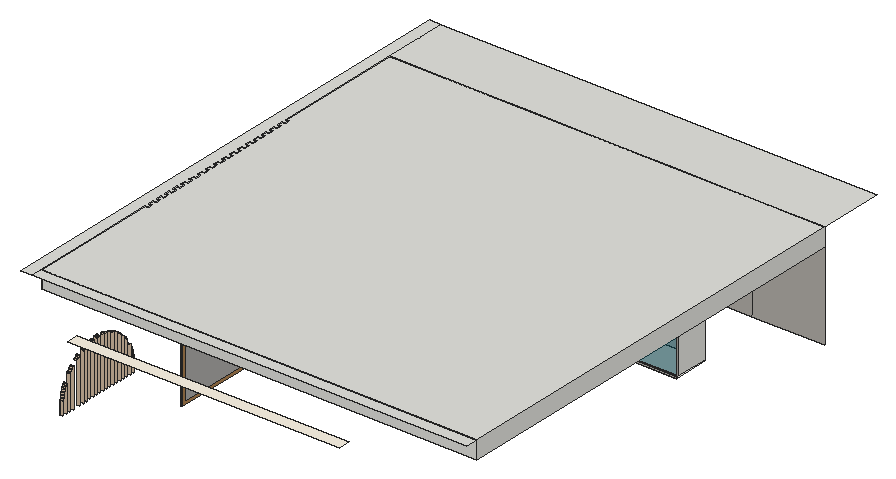
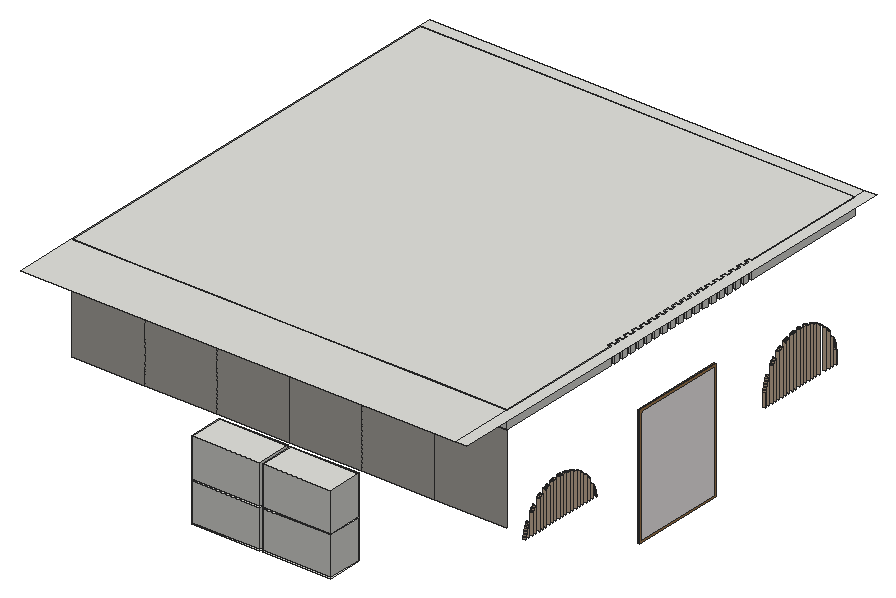
# SketchUp Ruby script. Lengths in inches.
U = 1.inch
M = Sketchup.active_model
def pt(a) = Geom::Point3d.new(a.map { |v| v * U })
def face(e, loops, mat)
  f = e.add_face(loops[0].map { |a| pt(a) })
  loops[1..].each { |l| e.add_face(l.map { |a| pt(a) }).erase! }
  f.material = f.back_material = mat if mat
  f
end
# faces: each face lists its corners as indices into pts; further lists are holes
def faces(e, pts, list, mat = nil) = list.each { |f| face(e, (f[0].is_a?(Array) ? f : [f]).map { |l| l.map { |i| pts[i] } }, mat) }
# xy, xz, yz: faces in a plane at the given z, y or x. An outline is a flat list of corners, or four numbers for a rectangle; further outlines are holes
def ring(l) = l.size == 4 ? [[l[0], l[1]], [l[2], l[1]], [l[2], l[3]], [l[0], l[3]]] : l.each_slice(2).to_a
def flat(e, list, mat, &to3) = list.each { |f| face(e, (f[0].is_a?(Array) ? f : [f]).map { |l| ring(l).map { |u, v| to3.(u, v) } }, mat) }
def xy(e, z, list, mat = nil) = flat(e, list, mat) { |x, y| [x, y, z] }
def xz(e, y, list, mat = nil) = flat(e, list, mat) { |x, z| [x, y, z] }
def yz(e, x, list, mat = nil) = flat(e, list, mat) { |y, z| [x, y, z] }
def lines(e, pts, list) = list.each { |a, b| e.add_line(pt(pts[a]), pt(pts[b])) }
# prism: a flat outline (further loops are holes) pulled along v
def prism(e, loops, v, mat = nil)
  f = face(e, loops, mat); d = Geom::Vector3d.new(v.map { |x| x * U })
  f.pushpull(f.normal.samedirection?(d) ? d.length : -d.length)
end
def box(e, o, s, mat = nil) = prism(e, [[o, [o[0] + s[0], o[1], o[2]], [o[0] + s[0], o[1] + s[1], o[2]], [o[0], o[1] + s[1], o[2]]]], [0, 0, s[2]], mat)
def at(x, y, z, deg = 0) = Geom::Transformation.translation(pt([x, y, z])) * Geom::Transformation.rotation(ORIGIN, Z_AXIS, deg.degrees)
def axes(o, x, y, z) = Geom::Transformation.new([*x, 0, *y, 0, *z, 0, *pt(o).to_a, 1])
def part(name) = M.definitions.add(name)
# library, detail: a bought-in or finely detailed component or shape, given as its bounding box
def library(name, o, s) = part(name).tap { |d| box(d.entities, o, s) }
def detail(e, o, s) = box(e.add_group.entities, o, s)
def put(e, d, t, mat = nil) = e.add_instance(d, t).tap { |i| i.material = mat if mat }
def group(e, t, mat = nil) = e.add_group.tap { |g| g.transformation = t; g.material = mat if mat }.entities
root = M.entities
M.materials.add("F15").color = [172, 171, 168]
M.materials.add("Querkus Oak Naturel Adagio _ Architonic1").color = [173, 130, 81]
M.materials.add("[0010_Snow]").color = [255, 250, 250]
M.materials.add("[0030_OldLace]").color = [253, 245, 230]
M.materials.add("[0052_FloralWhite]").color = [178, 175, 168]
M.materials.add("[0052_FloralWhite]1").color = [255, 250, 240]
M.materials.add("[Formica Laminate Light]").color = [213, 189, 164]
M.materials.add("[Translucent Glass Tinted]").color = [3, 85, 102]
M.materials["[Translucent Glass Tinted]"].alpha = 0.48
c1 = part("F7")
g1 = group(c1.entities,at(0,0,0))
xy(g1,0.5,[[0.5,0.3,18.5,0.6]])
xy(g1,24,[[0.5,0.3,18.5,0.6]])
xz(g1,0.3,[[0.5,0.5,18.5,24]],"F15")
xz(g1,0.6,[[0.5,0.5,18.5,24]],"[0010_Snow]")
yz(g1,0.5,[[0.3,0.5,0.6,24]])
yz(g1,18.5,[[0.3,0.5,0.6,24]])
g2 = group(g1,at(19,0,0),"Querkus Oak Naturel Adagio _ Architonic1")
prism(g2,[[[0,0.6,0],[0,0.6,24.5],[-19,0.6,24.5],[-19,0.6,0]],[[-0.5,0.6,0.5],[-18.5,0.6,0.5],[-18.5,0.6,24],[-0.5,0.6,24]]],[0,-0.6,0])
c2 = library("chandelier1 (1)",[151.15,151.6,16.88],[49.29,55.59,90.46])
xy(root,68.12,[[54.33,152.5,77.5,164],[78.5,152.5,101.67,164]])
xy(root,68.12,[[54.33,152,77.5,152.5],[78.5,152,101.67,152.5]],"[0052_FloralWhite]")
xy(root,68.62,[[54.33,152.5,77.5,164],[78.5,152.5,101.67,164]])
xy(root,68.62,[[54.33,152,77.5,152.5],[78.5,152,101.67,152.5]],"[0052_FloralWhite]")
xy(root,81.31,[[54.33,152.5,77.5,164],[78.5,152.5,101.67,164]])
xy(root,81.31,[[54.33,152,77.5,152.5],[78.5,152,101.67,152.5]],"[0052_FloralWhite]")
xy(root,81.81,[[54.33,152.5,77.5,164],[78.5,152.5,101.67,164]])
xy(root,81.81,[[54.33,152,77.5,152.5],[78.5,152,101.67,152.5]],"[0052_FloralWhite]")
xy(root,95,[[54.33,152.5,77.5,164],[78.5,152.5,101.67,164]])
xy(root,95,[[54.33,152,77.5,152.5],[78.5,152,101.67,152.5]],"[0052_FloralWhite]")
xy(root,101.71,[[4,24.84,5,24.86],[4,29.14,5,29.16],[4,126.84,5,126.86],[4,131.14,5,131.16]],"[Formica Laminate Light]")
xy(root,116.13,[[16.1875,0,108.6875,4]],"[0030_OldLace]")
xy(root,126,[[[4,4,4,48,5,48,5,49.71,4,49.71,4,51.43,5,51.43,5,53.14,4,53.14,4,54.86,5,54.86,5,56.57,4,56.57,4,58.29,5,58.29,5,60,4,60,4,61.71,5,61.71,5,63.43,4,63.43,4,65.14,5,65.14,5,66.86,4,66.86,4,68.57,5,68.57,5,70.29,4,70.29,4,72,5,72,5,73.71,4,73.71,4,75.43,5,75.43,5,77.14,4,77.14,4,78.86,5,78.86,5,80.57,4,80.57,4,82.29,5,82.29,5,84,4,84,4,85.71,5,85.71,5,87.43,4,87.43,4,89.14,5,89.14,5,90.86,4,90.86,4,92.57,5,92.57,5,94.29,4,94.29,4,96,5,96,5,97.71,4,97.71,4,99.43,5,99.43,5,101.14,4,101.14,4,102.86,5,102.86,5,104.57,4,104.57,4,106.29,5,106.29,5,108,4,108,4,152,152,152,152,4],[37.37,36.37,119.63,119.63]]],"[0052_FloralWhite]1")
xy(root,130,[[37.37,36.37,119.63,119.63]],"[0052_FloralWhite]1")
xy(root,132,[[0,0,4,0,4,48,5,48,5,49.71,4,49.71,4,51.43,5,51.43,5,53.14,4,53.14,4,54.86,5,54.86,5,56.57,4,56.57,4,58.29,5,58.29,5,60,4,60,4,61.71,5,61.71,5,63.43,4,63.43,4,65.14,5,65.14,5,66.86,4,66.86,4,68.57,5,68.57,5,70.29,4,70.29,4,72,5,72,5,73.71,4,73.71,4,75.43,5,75.43,5,77.14,4,77.14,4,78.86,5,78.86,5,80.57,4,80.57,4,82.29,5,82.29,5,84,4,84,4,85.71,5,85.71,5,87.43,4,87.43,4,89.14,5,89.14,5,90.86,4,90.86,4,92.57,5,92.57,5,94.29,4,94.29,4,96,5,96,5,97.71,4,97.71,4,99.43,5,99.43,5,101.14,4,101.14,4,102.86,5,102.86,5,104.57,4,104.57,4,106.29,5,106.29,5,108,4,108,4,174,0,174],[4,0,152,4],[4,4,152,4,152,152,4,152,4,108,5,108,5,106.29,4,106.29,4,104.57,5,104.57,5,102.86,4,102.86,4,101.14,5,101.14,5,99.43,4,99.43,4,97.71,5,97.71,5,96,4,96,4,94.29,5,94.29,5,92.57,4,92.57,4,90.86,5,90.86,5,89.14,4,89.14,4,87.43,5,87.43,5,85.71,4,85.71,4,84,5,84,5,82.29,4,82.29,4,80.57,5,80.57,5,78.86,4,78.86,4,77.14,5,77.14,5,75.43,4,75.43,4,73.71,5,73.71,5,72,4,72,4,70.29,5,70.29,5,68.57,4,68.57,4,66.86,5,66.86,5,65.14,4,65.14,4,63.43,5,63.43,5,61.71,4,61.71,4,60,5,60,5,58.29,4,58.29,4,56.57,5,56.57,5,54.86,4,54.86,4,53.14,5,53.14,5,51.43,4,51.43,4,49.71,5,49.71,5,48,4,48],[4,152,152,174]])
xz(root,4,[[4,126,152,132]])
xz(root,12,[[4,84.25,5,88.86]],"[Formica Laminate Light]")
xz(root,13.43,[[4,84.25,5,93.49]],"[Formica Laminate Light]")
xz(root,14.86,[[4,84.25,5,95.8]],"[Formica Laminate Light]")
xz(root,16.29,[[4,84.25,5,97.4375]],"[Formica Laminate Light]")
xz(root,19.14,[[4,84.25,5,99.67]],"[Formica Laminate Light]")
xz(root,20.57,[[4,84.25,5,100.43]],"[Formica Laminate Light]")
xz(root,22,[[4,84.25,5,101.01]],"[Formica Laminate Light]")
xz(root,23.43,[[4,84.25,5,101.43]],"[Formica Laminate Light]")
xz(root,24.86,[[4,84.25,5,101.71]],"[Formica Laminate Light]")
xz(root,26.29,[[4,84.25,5,101.84]],"[Formica Laminate Light]")
xz(root,27.71,[[4,84.25,5,101.84]],"[Formica Laminate Light]")
xz(root,29.14,[[4,84.25,5,101.71]],"[Formica Laminate Light]")
xz(root,30.57,[[4,84.25,5,101.43]],"[Formica Laminate Light]")
xz(root,32,[[4,84.25,5,101.01]],"[Formica Laminate Light]")
xz(root,33.43,[[4,84.25,5,100.43]],"[Formica Laminate Light]")
xz(root,34.86,[[4,84.25,5,99.67]],"[Formica Laminate Light]")
xz(root,36.29,[[4,84.25,5,98.69]],"[Formica Laminate Light]")
xz(root,36.37,[[37.37,126,119.63,130]],"[0052_FloralWhite]1")
xz(root,37.71,[[4,84.25,5,97.4375]],"[Formica Laminate Light]")
xz(root,39.14,[[4,84.25,5,95.8]],"[Formica Laminate Light]")
xz(root,40.57,[[4,84.25,5,93.49]],"[Formica Laminate Light]")
xz(root,42,[[4,84.25,5,88.86]],"[Formica Laminate Light]")
xz(root,48,[[4,126,5,132]])
xz(root,49.71,[[4,126,5,132]])
xz(root,51.43,[[4,126,5,132]])
xz(root,53.14,[[4,126,5,132]])
xz(root,54.86,[[4,126,5,132]])
xz(root,56.57,[[4,126,5,132]])
xz(root,58.29,[[4,126,5,132]])
xz(root,60,[[4,126,5,132]])
xz(root,61.71,[[4,126,5,132]])
xz(root,63.43,[[4,126,5,132]])
xz(root,65.14,[[4,126,5,132]])
xz(root,66.86,[[4,126,5,132]])
xz(root,68.57,[[4,126,5,132]])
xz(root,70.29,[[4,126,5,132]])
xz(root,72,[[4,126,5,132]])
xz(root,73.71,[[4,126,5,132]])
xz(root,75.43,[[4,126,5,132]])
xz(root,77.14,[[4,126,5,132]])
xz(root,78.86,[[4,126,5,132]])
xz(root,80.57,[[4,126,5,132]])
xz(root,82.29,[[4,126,5,132]])
xz(root,84,[[4,126,5,132]])
xz(root,85.71,[[4,126,5,132]])
xz(root,87.43,[[4,126,5,132]])
xz(root,89.14,[[4,126,5,132]])
xz(root,90.86,[[4,126,5,132]])
xz(root,92.57,[[4,126,5,132]])
xz(root,94.29,[[4,126,5,132]])
xz(root,96,[[4,126,5,132]])
xz(root,97.71,[[4,126,5,132]])
xz(root,99.43,[[4,126,5,132]])
xz(root,101.14,[[4,126,5,132]])
xz(root,102.86,[[4,126,5,132]])
xz(root,104.57,[[4,126,5,132]])
xz(root,106.29,[[4,126,5,132]])
xz(root,108,[[4,126,5,132]])
xz(root,115.43,[[4,88.86,5,93.49]],"[Formica Laminate Light]")
xz(root,116.86,[[4,88.86,5,95.8]],"[Formica Laminate Light]")
xz(root,118.29,[[4,88.86,5,97.4375]],"[Formica Laminate Light]")
xz(root,119.63,[[37.37,126,119.63,130]],"[0052_FloralWhite]1")
xz(root,119.71,[[4,88.86,5,98.69]],"[Formica Laminate Light]")
xz(root,121.14,[[4,88.86,5,99.67]],"[Formica Laminate Light]")
xz(root,122.57,[[4,88.86,5,100.43]],"[Formica Laminate Light]")
xz(root,124,[[4,88.86,5,101.01]],"[Formica Laminate Light]")
xz(root,125.43,[[4,88.86,5,101.43]],"[Formica Laminate Light]")
xz(root,126.86,[[4,88.86,5,101.71]],"[Formica Laminate Light]")
xz(root,128.29,[[4,88.86,5,101.84]],"[Formica Laminate Light]")
xz(root,129.71,[[4,88.86,5,101.84]],"[Formica Laminate Light]")
xz(root,131.14,[[4,88.86,5,101.71]],"[Formica Laminate Light]")
xz(root,132.57,[[4,88.86,5,101.43]],"[Formica Laminate Light]")
xz(root,134,[[4,88.86,5,101.01]],"[Formica Laminate Light]")
xz(root,135.43,[[4,88.86,5,100.43]],"[Formica Laminate Light]")
xz(root,136.86,[[4,88.86,5,99.67]],"[Formica Laminate Light]")
xz(root,138.29,[[4,88.86,5,98.69]],"[Formica Laminate Light]")
xz(root,139.71,[[4,88.86,5,97.4375]],"[Formica Laminate Light]")
xz(root,141.14,[[4,88.86,5,95.8]],"[Formica Laminate Light]")
xz(root,142.57,[[4,88.86,5,93.49]],"[Formica Laminate Light]")
xz(root,152,[[4,126,28.67,132],[28.67,126,53.33,132],[53.33,126,78,132],[78,126,102.67,132],[102.67,126,127.33,132],
  [127.33,126,152,132]])
xz(root,152,[[54.33,68.12,77.5,68.62],[78.5,68.12,101.67,68.62],[54.33,81.31,77.5,81.81],[78.5,81.31,101.67,81.81],[4,96,28.67,126],
  [28.67,96,53.33,126],[53.33,96,78,126],[78,96,102.67,126],[102.67,96,127.33,126],[127.33,96,152,126]],"[0052_FloralWhite]")
xz(root,152.5,[[54.33,68.62,77.5,81.31],[78.5,68.62,101.67,81.31],[54.33,81.81,77.5,95],[78.5,81.81,101.67,95]],"[Translucent Glass Tinted]")
xz(root,164,[[54.33,68.62,77.5,81.31],[78.5,68.62,101.67,81.31],[54.33,81.81,77.5,95],[78.5,81.81,101.67,95]])
yz(root,4,[[12,84.25,12,88.86,11.93,88.62],[42,84.25,42.07,88.62,42,88.86],[4,126,48,132],[49.71,126,51.43,132],[53.14,126,54.86,132],
  [56.57,126,58.29,132],[60,126,61.71,132],[63.43,126,65.14,132],[66.86,126,68.57,132],[70.29,126,72,132],
  [73.71,126,75.43,132],[77.14,126,78.86,132],[80.57,126,82.29,132],[84,126,85.71,132],[87.43,126,89.14,132],
  [90.86,126,92.57,132],[94.29,126,96,132],[97.71,126,99.43,132],[101.14,126,102.86,132],[104.57,126,106.29,132],
  [108,126,152,132]])
yz(root,5,[[48,126,49.71,132],[51.43,126,53.14,132],[54.86,126,56.57,132],[58.29,126,60,132],[61.71,126,63.43,132],
  [65.14,126,66.86,132],[68.57,126,70.29,132],[72,126,73.71,132],[75.43,126,77.14,132],[78.86,126,80.57,132],
  [82.29,126,84,132],[85.71,126,87.43,132],[89.14,126,90.86,132],[92.57,126,94.29,132],[96,126,97.71,132],
  [99.43,126,101.14,132],[102.86,126,104.57,132],[106.29,126,108,132]])
yz(root,37.37,[[36.37,126,119.63,130]],"[0052_FloralWhite]1")
yz(root,54.33,[[152,68.12,152.5,68.62],[152.5,68.62,164,81.31],[152,81.31,152.5,81.81],[152.5,81.81,164,95]])
yz(root,54.33,[[152,68.62,152.5,81.31],[152,81.81,152.5,95]],"[0052_FloralWhite]")
yz(root,77.5,[[152.5,68.62,164,81.31],[152.5,81.81,164,95]])
yz(root,77.5,[[152,68.62,152.5,81.31],[152,81.81,152.5,95]],"[0052_FloralWhite]")
yz(root,78.5,[[152.5,68.62,164,81.31],[152.5,81.81,164,95]])
yz(root,78.5,[[152,68.62,152.5,81.31],[152,81.81,152.5,95]],"[0052_FloralWhite]")
yz(root,101.67,[[152.5,68.62,164,81.31],[152.5,81.81,164,95]])
yz(root,101.67,[[152,68.62,152.5,81.31],[152,81.81,152.5,95]],"[0052_FloralWhite]")
yz(root,119.63,[[36.37,126,119.63,130]],"[0052_FloralWhite]1")
yz(root,152,[[4,126,152,132]])
p = [[4,12.04,89.29],[4,12,88.86],[5,12,88.86],[5,12.04,89.29],[4,42,88.86],[4,41.96,89.29],
  [5,41.96,89.29],[5,42,88.86],[4,114.04,89.29],[4,114,88.86],[5,114,88.86],[5,114.04,89.29],
  [4,144,88.86],[4,143.96,89.29],[5,143.96,89.29],[5,144,88.86],[4,12.12,89.72],[5,12.12,89.72],
  [4,41.88,89.72],[5,41.88,89.72],[4,114.12,89.72],[5,114.12,89.72],[4,143.88,89.72],[5,143.88,89.72],
  [4,12.21,90.14],[5,12.21,90.14],[4,41.79,90.14],[5,41.79,90.14],[4,114.21,90.14],[5,114.21,90.14],
  [4,143.79,90.14],[5,143.79,90.14],[4,12.3125,90.5625],[5,12.3125,90.5625],[4,41.6875,90.5625],[5,41.6875,90.5625],
  [4,114.3125,90.5625],[5,114.3125,90.5625],[4,143.6875,90.5625],[5,143.6875,90.5625],[4,12.43,90.98],[5,12.43,90.98],
  [4,41.57,90.98],[5,41.57,90.98],[4,114.43,90.98],[5,114.43,90.98],[4,143.57,90.98],[5,143.57,90.98],
  [4,12.56,91.39],[5,12.56,91.39],[4,41.44,91.39],[5,41.44,91.39],[4,114.56,91.39],[5,114.56,91.39],
  [4,143.44,91.39],[5,143.44,91.39],[4,12.7,91.8],[5,12.7,91.8],[4,41.3,91.8],[5,41.3,91.8],
  [4,114.7,91.8],[5,114.7,91.8],[4,143.3,91.8],[5,143.3,91.8],[4,12.85,92.21],[5,12.85,92.21],
  [4,41.15,92.21],[5,41.15,92.21],[4,114.85,92.21],[5,114.85,92.21],[4,143.15,92.21],[5,143.15,92.21],
  [4,13.02,92.61],[5,13.02,92.61],[4,40.98,92.61],[5,40.98,92.61],[4,115.02,92.61],[5,115.02,92.61],
  [4,142.98,92.61],[5,142.98,92.61],[4,13.19,93],[5,13.19,93],[4,40.81,93],[5,40.81,93],
  [4,115.19,93],[5,115.19,93],[4,142.81,93],[5,142.81,93],[4,13.38,93.4],[5,13.38,93.4],
  [4,40.62,93.4],[5,40.62,93.4],[4,115.38,93.4],[5,115.38,93.4],[4,142.62,93.4],[5,142.62,93.4],
  [4,13.43,93.49],[5,13.43,93.49],[4,40.57,93.49],[5,40.57,93.49],[4,115.43,93.49],[5,115.43,93.49],
  [4,142.57,93.49],[5,142.57,93.49],[4,14.98,95.96],[4,14.86,95.8],[5,14.86,95.8],[5,14.98,95.96],
  [4,39.14,95.8],[4,39.02,95.96],[5,39.02,95.96],[5,39.14,95.8],[4,116.98,95.96],[4,116.86,95.8],
  [5,116.86,95.8],[5,116.98,95.96],[4,141.14,95.8],[4,141.02,95.96],[5,141.02,95.96],[5,141.14,95.8],
  [4,15.25,96.3],[5,15.25,96.3],[4,38.75,96.3],[5,38.75,96.3],[4,117.25,96.3],[5,117.25,96.3],
  [4,140.75,96.3],[5,140.75,96.3],[4,15.53,96.63],[5,15.53,96.63],[4,38.47,96.63],[5,38.47,96.63],
  [4,117.53,96.63],[5,117.53,96.63],[4,140.47,96.63],[5,140.47,96.63],[4,15.82,96.96],[5,15.82,96.96],
  [4,38.18,96.96],[5,38.18,96.96],[4,117.82,96.96],[5,117.82,96.96],[4,140.18,96.96],[5,140.18,96.96],
  [4,16.12,97.27],[5,16.12,97.27],[4,37.88,97.27],[5,37.88,97.27],[4,118.12,97.27],[5,118.12,97.27],
  [4,139.88,97.27],[5,139.88,97.27],[4,16.29,97.4375],[5,16.29,97.4375],[4,37.71,97.4375],[5,37.71,97.4375],
  [4,118.29,97.4375],[5,118.29,97.4375],[4,139.71,97.4375],[5,139.71,97.4375],[4,17.73,98.71],[4,17.71,98.69],
  [5,17.71,98.69],[5,17.73,98.71],[4,18.08,98.97],[5,18.08,98.97],[4,36.27,98.71],[4,35.92,98.97],
  [5,35.92,98.97],[5,36.27,98.71],[4,36.29,98.69],[5,36.29,98.69],[4,119.73,98.71],[4,119.71,98.69],
  [5,119.71,98.69],[5,119.73,98.71],[4,120.08,98.97],[5,120.08,98.97],[4,138.27,98.71],[4,137.92,98.97],
  [5,137.92,98.97],[5,138.27,98.71],[4,138.29,98.69],[5,138.29,98.69],[4,18.4375,99.22],[5,18.4375,99.22],
  [4,35.5625,99.22],[5,35.5625,99.22],[4,120.4375,99.22],[5,120.4375,99.22],[4,137.5625,99.22],[5,137.5625,99.22],
  [4,18.8,99.46],[5,18.8,99.46],[4,35.2,99.46],[5,35.2,99.46],[4,120.8,99.46],[5,120.8,99.46],
  [4,137.2,99.46],[5,137.2,99.46],[4,19.14,99.67],[5,19.14,99.67],[4,34.86,99.67],[5,34.86,99.67],
  [4,121.14,99.67],[5,121.14,99.67],[4,136.86,99.67],[5,136.86,99.67],[4,20.7,100.49],[4,20.57,100.43],
  [5,20.57,100.43],[5,20.7,100.49],[4,33.43,100.43],[4,33.3,100.49],[5,33.3,100.49],[5,33.43,100.43],
  [4,122.7,100.49],[4,122.57,100.43],[5,122.57,100.43],[5,122.7,100.49],[4,135.43,100.43],[4,135.3,100.49],
  [5,135.3,100.49],[5,135.43,100.43],[4,21.09,100.67],[5,21.09,100.67],[4,32.91,100.67],[5,32.91,100.67],
  [4,123.09,100.67],[5,123.09,100.67],[4,134.91,100.67],[5,134.91,100.67],[4,21.5,100.83],[5,21.5,100.83],
  [4,32.5,100.83],[5,32.5,100.83],[4,123.5,100.83],[5,123.5,100.83],[4,134.5,100.83],[5,134.5,100.83],
  [4,21.9,100.98],[5,21.9,100.98],[4,32.1,100.98],[5,32.1,100.98],[4,123.9,100.98],[5,123.9,100.98],
  [4,134.1,100.98],[5,134.1,100.98],[4,22,101.01],[5,22,101.01],[4,32,101.01],[5,32,101.01],
  [4,124,101.01],[5,124,101.01],[4,134,101.01],[5,134,101.01],[4,23.5625,101.47],[4,23.43,101.43],
  [5,23.43,101.43],[5,23.5625,101.47],[4,30.57,101.43],[4,30.4375,101.47],[5,30.4375,101.47],[5,30.57,101.43],
  [4,125.5625,101.47],[4,125.43,101.43],[5,125.43,101.43],[5,125.5625,101.47],[4,132.57,101.43],[4,132.4375,101.47],
  [5,132.4375,101.47],[5,132.57,101.43],[4,23.99,101.56],[5,23.99,101.56],[4,30.01,101.56],[5,30.01,101.56],
  [4,125.99,101.56],[5,125.99,101.56],[4,132.01,101.56],[5,132.01,101.56],[4,24.41,101.64],[5,24.41,101.64],
  [4,24.84,101.71],[5,24.84,101.71],[4,29.59,101.64],[4,29.16,101.71],[5,29.16,101.71],[5,29.59,101.64],
  [4,126.41,101.64],[5,126.41,101.64],[4,126.84,101.71],[5,126.84,101.71],[4,131.59,101.64],[4,131.16,101.71],
  [5,131.16,101.71],[5,131.59,101.64],[4,26.57,101.85],[4,26.29,101.84],[5,26.29,101.84],[5,26.57,101.85],
  [4,27.71,101.84],[4,27.43,101.85],[5,27.43,101.85],[5,27.71,101.84],[4,128.57,101.85],[4,128.29,101.84],
  [5,128.29,101.84],[5,128.57,101.85],[4,129.71,101.84],[4,129.43,101.85],[5,129.43,101.85],[5,129.71,101.84],
  [4,27,101.86],[5,27,101.86],[4,129,101.86],[5,129,101.86]]
faces(root,p,[[0,1,2,3],[4,5,6,7],[8,9,10,11],[12,13,14,15],[16,0,3,17],[5,18,19,6],[20,8,11,21],[13,22,23,14],
  [24,16,17,25],[18,26,27,19],[28,20,21,29],[22,30,31,23],[32,24,25,33],[26,34,35,27],[36,28,29,37],[30,38,39,31],
  [40,32,33,41],[34,42,43,35],[44,36,37,45],[38,46,47,39],[48,40,41,49],[42,50,51,43],[52,44,45,53],[46,54,55,47],
  [56,48,49,57],[50,58,59,51],[60,52,53,61],[54,62,63,55],[64,56,57,65],[58,66,67,59],[68,60,61,69],[62,70,71,63],
  [72,64,65,73],[66,74,75,67],[76,68,69,77],[70,78,79,71],[80,72,73,81],[74,82,83,75],[84,76,77,85],[78,86,87,79],
  [88,80,81,89],[82,90,91,83],[92,84,85,93],[86,94,95,87],[96,88,89,97],[90,98,99,91],[100,92,93,101],[94,102,103,95],
  [104,105,106,107],[108,109,110,111],[112,113,114,115],[116,117,118,119],[120,104,107,121],[109,122,123,110],[124,112,115,125],[117,126,127,118],
  [128,120,121,129],[122,130,131,123],[132,124,125,133],[126,134,135,127],[136,128,129,137],[130,138,139,131],[140,132,133,141],[134,142,143,135],
  [144,136,137,145],[138,146,147,139],[148,140,141,149],[142,150,151,143],[152,144,145,153],[146,154,155,147],[156,148,149,157],[150,158,159,151],
  [160,161,162,163],[164,160,163,165],[166,167,168,169],[170,166,169,171],[172,173,174,175],[176,172,175,177],[178,179,180,181],[182,178,181,183],
  [184,164,165,185],[167,186,187,168],[188,176,177,189],[179,190,191,180],[192,184,185,193],[186,194,195,187],[196,188,189,197],[190,198,199,191],
  [200,192,193,201],[194,202,203,195],[204,196,197,205],[198,206,207,199],[208,209,210,211],[212,213,214,215],[216,217,218,219],[220,221,222,223],
  [224,208,211,225],[213,226,227,214],[228,216,219,229],[221,230,231,222],[232,224,225,233],[226,234,235,227],[236,228,229,237],[230,238,239,231],
  [240,232,233,241],[234,242,243,235],[244,236,237,245],[238,246,247,239],[248,240,241,249],[242,250,251,243],[252,244,245,253],[246,254,255,247],
  [256,257,258,259],[260,261,262,263],[264,265,266,267],[268,269,270,271],[272,256,259,273],[261,274,275,262],[276,264,267,277],[269,278,279,270],
  [280,272,273,281],[282,280,281,283],[284,285,286,287],[274,284,287,275],[288,276,277,289],[290,288,289,291],[292,293,294,295],[278,292,295,279],
  [296,297,298,299],[300,301,302,303],[304,305,306,307],[308,309,310,311],[312,296,299,313],[301,312,313,302],[314,304,307,315],[309,314,315,310]],"[Formica Laminate Light]")
put(root,c1,axes([5.6,61.9375,65.46],[0,1.70256,0],[-1,0,0],[0,0,1.6616]))
put(root,c2,axes([-9.47,9.01,103.17],[0.5,0,0],[0,0.38551,0],[0,0,0.25]))
